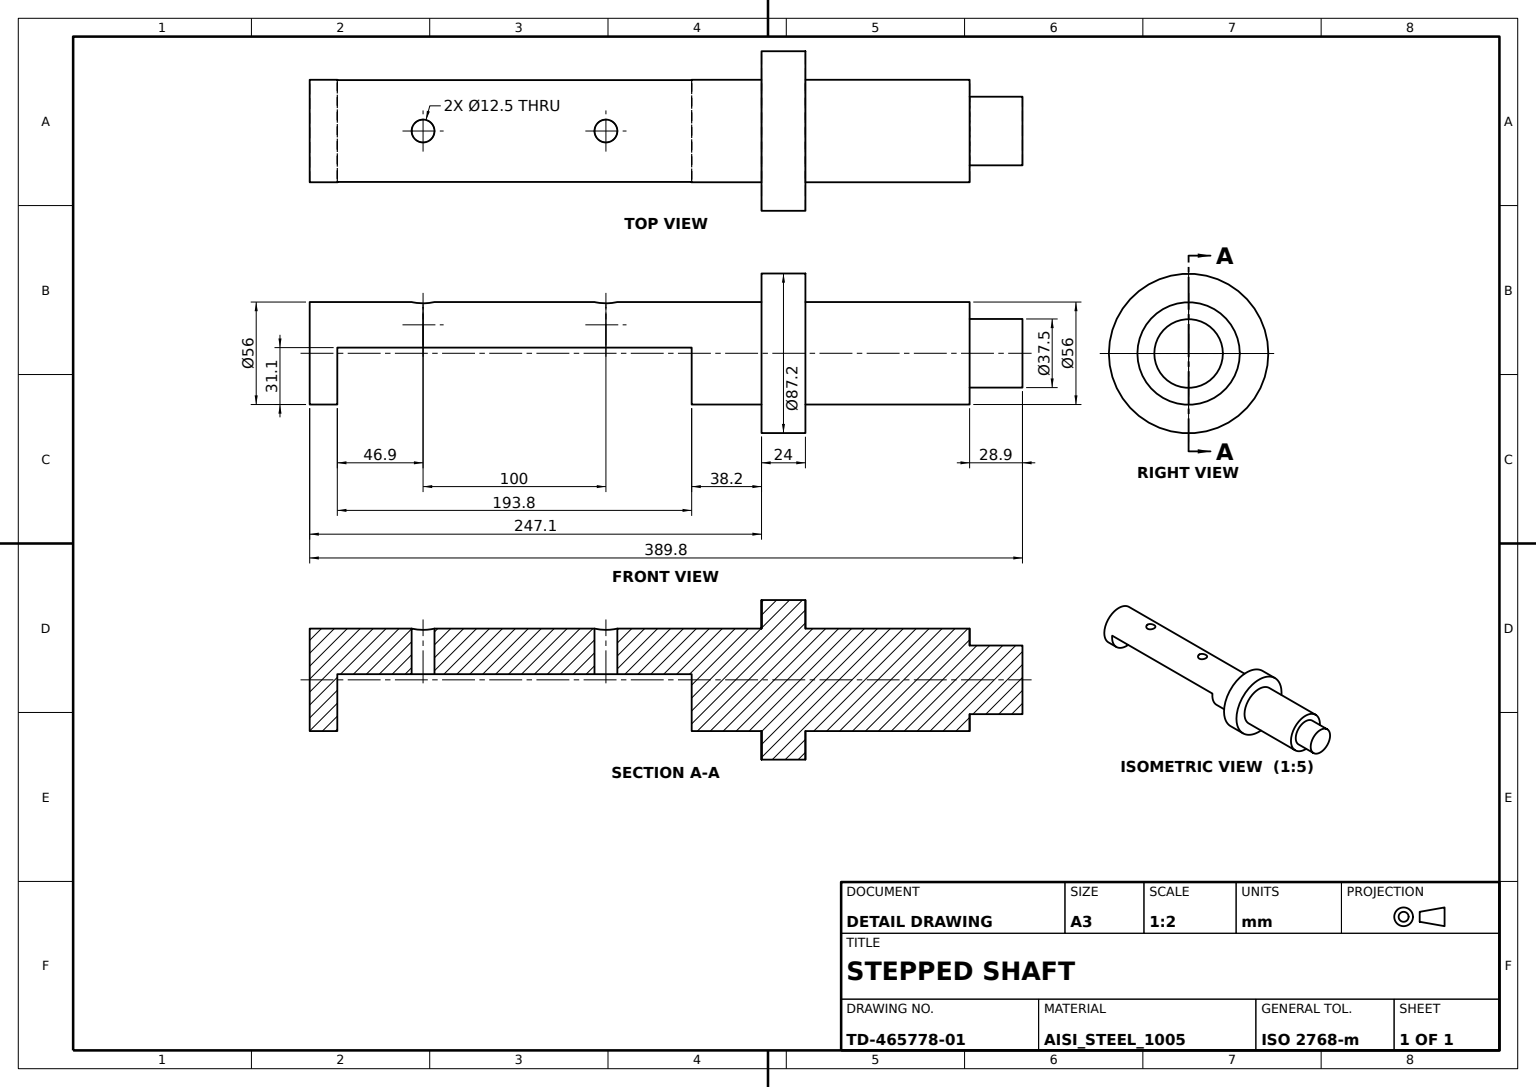
ISO-10303-21;
HEADER;
FILE_DESCRIPTION((''),'2;1');
FILE_NAME('','',(''),(''),'','','');
FILE_SCHEMA(('AUTOMOTIVE_DESIGN'));
ENDSEC;
DATA;
#1=APPLICATION_CONTEXT('');
#2=PRODUCT_CONTEXT('',#1,'mechanical');
#3=PRODUCT('','','',(#2));
#4=PRODUCT_DEFINITION_FORMATION('','',#3);
#5=PRODUCT_DEFINITION_CONTEXT('',#1,'design');
#6=PRODUCT_DEFINITION('','',#4,#5);
#7=PRODUCT_DEFINITION_SHAPE('','',#6);
#8=(LENGTH_UNIT()NAMED_UNIT(*)SI_UNIT(.MILLI.,.METRE.));
#9=(NAMED_UNIT(*)PLANE_ANGLE_UNIT()SI_UNIT($,.RADIAN.));
#10=(NAMED_UNIT(*)SI_UNIT($,.STERADIAN.)SOLID_ANGLE_UNIT());
#11=UNCERTAINTY_MEASURE_WITH_UNIT(LENGTH_MEASURE(0.005),#8,'distance_accuracy_value','');
#12=(GEOMETRIC_REPRESENTATION_CONTEXT(3)GLOBAL_UNCERTAINTY_ASSIGNED_CONTEXT((#11))GLOBAL_UNIT_ASSIGNED_CONTEXT((#8,#9,#10))REPRESENTATION_CONTEXT('',''));
#13=CARTESIAN_POINT('',(0.,18.75,142.7));
#14=VERTEX_POINT('',#13);
#15=CARTESIAN_POINT('',(0.,0.,142.7));
#16=DIRECTION('',(0.,0.,1.));
#17=DIRECTION('',(0.,1.,0.));
#18=AXIS2_PLACEMENT_3D('',#15,#16,#17);
#19=CIRCLE('',#18,18.75);
#20=EDGE_CURVE('',#14,#14,#19,.T.);
#21=ORIENTED_EDGE('',*,*,#20,.T.);
#22=EDGE_LOOP('',(#21));
#23=FACE_BOUND('',#22,.T.);
#24=DIRECTION('',(1.,0.,0.));
#25=AXIS2_PLACEMENT_3D('',#15,#16,#24);
#26=PLANE('',#25);
#27=ADVANCED_FACE('',(#23),#26,.T.);
#28=CARTESIAN_POINT('',(-28.,0.,-191.35));
#29=VERTEX_POINT('',#28);
#30=CARTESIAN_POINT('',(-27.923292,-2.470226,-191.018368));
#31=CARTESIAN_POINT('',(-28.038226,0.001909,-191.51522));
#32=CARTESIAN_POINT('',(-27.923806,2.462591,-191.020753));
#33=CARTESIAN_POINT('',(-27.649413,4.534425,-189.632288));
#34=CARTESIAN_POINT('',(-27.371989,5.92072,-187.562091));
#35=CARTESIAN_POINT('',(-27.254483,6.413877,-185.104449));
#36=CARTESIAN_POINT('',(-27.37134,5.923765,-182.643032));
#37=CARTESIAN_POINT('',(-27.649543,4.533953,-180.566538));
#38=CARTESIAN_POINT('',(-27.923952,2.461325,-179.178709));
#39=CARTESIAN_POINT('',(-28.037916,0.002745,-178.686152));
#40=CARTESIAN_POINT('',(-27.924382,-2.456758,-179.176687));
#41=CARTESIAN_POINT('',(-27.650228,-4.529699,-180.56301));
#42=CARTESIAN_POINT('',(-27.372311,-5.919433,-182.633271));
#43=CARTESIAN_POINT('',(-27.254354,-6.414385,-185.096275));
#44=CARTESIAN_POINT('',(-27.371534,-5.923021,-187.558096));
#45=CARTESIAN_POINT('',(-27.649072,-4.535591,-189.63023));
#46=B_SPLINE_CURVE_WITH_KNOTS('',3,(#30,#31,#32,#33,#34,#35,#36,#37,#38,#39,#40,#41,#42,#43,#44,#45,#30,#31,#32),.UNSPECIFIED.,.T.,.F.,(1,1,1,1,1,1,1,1,1,1,1,1,1,1,1,1,1,1,1,1,1,1,1),(-0.00734987,-0.004899913,-0.002449957,0.,0.002449957,0.004899913,0.00734987,0.009799826,0.012249783,0.014699739,0.017149696,0.019599653,0.022049609,0.024499566,0.026949522,0.029399479,0.031849436,0.034299392,0.036749349,0.039199305,0.041649262,0.044099218,0.046549175),.UNSPECIFIED.);
#47=EDGE_CURVE('',#29,#29,#46,.T.);
#48=ORIENTED_EDGE('',*,*,#47,.F.);
#49=EDGE_LOOP('',(#48));
#50=FACE_BOUND('',#49,.T.);
#51=CARTESIAN_POINT('',(-3.1,0.,-178.85));
#52=VERTEX_POINT('',#51);
#53=CARTESIAN_POINT('',(-3.1,0.,-185.1));
#54=AXIS2_PLACEMENT_3D('',#53,#24,#16);
#55=CIRCLE('',#54,6.25);
#56=EDGE_CURVE('',#52,#52,#55,.T.);
#57=ORIENTED_EDGE('',*,*,#56,.T.);
#58=EDGE_LOOP('',(#57));
#59=FACE_BOUND('',#58,.T.);
#60=CARTESIAN_POINT('',(-47.65,0.,-185.1));
#61=DIRECTION('',(0.,0.,-1.));
#62=AXIS2_PLACEMENT_3D('',#60,#24,#61);
#63=CYLINDRICAL_SURFACE('',#62,6.25);
#64=ADVANCED_FACE('',(#50,#59),#63,.F.);
#65=CARTESIAN_POINT('',(0.,18.75,113.8));
#66=VERTEX_POINT('',#65);
#67=CARTESIAN_POINT('',(0.,0.,113.8));
#68=AXIS2_PLACEMENT_3D('',#67,#16,#17);
#69=CIRCLE('',#68,18.75);
#70=EDGE_CURVE('',#66,#66,#69,.T.);
#71=ORIENTED_EDGE('',*,*,#70,.F.);
#72=EDGE_LOOP('',(#71));
#73=FACE_BOUND('',#72,.T.);
#74=CARTESIAN_POINT('',(0.,28.,113.8));
#75=VERTEX_POINT('',#74);
#76=CIRCLE('',#68,28.);
#77=EDGE_CURVE('',#75,#75,#76,.T.);
#78=ORIENTED_EDGE('',*,*,#77,.T.);
#79=EDGE_LOOP('',(#78));
#80=FACE_BOUND('',#79,.T.);
#81=AXIS2_PLACEMENT_3D('',#67,#16,#24);
#82=PLANE('',#81);
#83=ADVANCED_FACE('',(#73,#80),#82,.T.);
#84=CARTESIAN_POINT('',(0.,28.,24.));
#85=VERTEX_POINT('',#84);
#86=CARTESIAN_POINT('',(0.,0.,24.));
#87=AXIS2_PLACEMENT_3D('',#86,#16,#17);
#88=CIRCLE('',#87,28.);
#89=EDGE_CURVE('',#85,#85,#88,.T.);
#90=ORIENTED_EDGE('',*,*,#89,.F.);
#91=EDGE_LOOP('',(#90));
#92=FACE_BOUND('',#91,.T.);
#93=CARTESIAN_POINT('',(0.,43.6,24.));
#94=VERTEX_POINT('',#93);
#95=CIRCLE('',#87,43.6);
#96=EDGE_CURVE('',#94,#94,#95,.T.);
#97=ORIENTED_EDGE('',*,*,#96,.T.);
#98=EDGE_LOOP('',(#97));
#99=FACE_BOUND('',#98,.T.);
#100=AXIS2_PLACEMENT_3D('',#86,#16,#24);
#101=PLANE('',#100);
#102=ADVANCED_FACE('',(#92,#99),#101,.T.);
#103=ORIENTED_EDGE('',*,*,#96,.F.);
#104=EDGE_LOOP('',(#103));
#105=FACE_BOUND('',#104,.T.);
#106=CARTESIAN_POINT('',(0.,43.6,0.));
#107=VERTEX_POINT('',#106);
#108=CARTESIAN_POINT('',(0.,0.,0.));
#109=AXIS2_PLACEMENT_3D('',#108,#16,#17);
#110=CIRCLE('',#109,43.6);
#111=EDGE_CURVE('',#107,#107,#110,.T.);
#112=ORIENTED_EDGE('',*,*,#111,.T.);
#113=EDGE_LOOP('',(#112));
#114=FACE_BOUND('',#113,.T.);
#115=DIRECTION('',(-1.,0.,0.));
#116=AXIS2_PLACEMENT_3D('',#86,#61,#115);
#117=CYLINDRICAL_SURFACE('',#116,43.6);
#118=ADVANCED_FACE('',(#105,#114),#117,.T.);
#119=ORIENTED_EDGE('',*,*,#70,.T.);
#120=EDGE_LOOP('',(#119));
#121=FACE_BOUND('',#120,.T.);
#122=ORIENTED_EDGE('',*,*,#20,.F.);
#123=EDGE_LOOP('',(#122));
#124=FACE_BOUND('',#123,.T.);
#125=AXIS2_PLACEMENT_3D('',#15,#61,#115);
#126=CYLINDRICAL_SURFACE('',#125,18.75);
#127=ADVANCED_FACE('',(#121,#124),#126,.T.);
#128=ORIENTED_EDGE('',*,*,#77,.F.);
#129=EDGE_LOOP('',(#128));
#130=FACE_BOUND('',#129,.T.);
#131=ORIENTED_EDGE('',*,*,#89,.T.);
#132=EDGE_LOOP('',(#131));
#133=FACE_BOUND('',#132,.T.);
#134=AXIS2_PLACEMENT_3D('',#67,#61,#115);
#135=CYLINDRICAL_SURFACE('',#134,28.);
#136=ADVANCED_FACE('',(#130,#133),#135,.T.);
#137=CARTESIAN_POINT('',(-3.1,-27.827864,-232.));
#138=VERTEX_POINT('',#137);
#139=CARTESIAN_POINT('',(-3.1,27.827864,-232.));
#140=VERTEX_POINT('',#139);
#141=CARTESIAN_POINT('',(0.,0.,-232.));
#142=AXIS2_PLACEMENT_3D('',#141,#61,#115);
#143=CIRCLE('',#142,28.);
#144=EDGE_CURVE('',#138,#140,#143,.F.);
#145=ORIENTED_EDGE('',*,*,#144,.T.);
#146=CARTESIAN_POINT('',(-3.1,28.9,-232.));
#147=DIRECTION('',(0.,-1.,0.));
#148=VECTOR('',#147,1000.);
#149=LINE('',#146,#148);
#150=EDGE_CURVE('',#138,#140,#149,.F.);
#151=ORIENTED_EDGE('',*,*,#150,.F.);
#152=EDGE_LOOP('',(#145,#151));
#153=FACE_BOUND('',#152,.T.);
#154=AXIS2_PLACEMENT_3D('',#146,#61,#115);
#155=PLANE('',#154);
#156=ADVANCED_FACE('',(#153),#155,.F.);
#157=CARTESIAN_POINT('',(0.,28.,-247.1));
#158=VERTEX_POINT('',#157);
#159=CARTESIAN_POINT('',(0.,0.,-247.1));
#160=AXIS2_PLACEMENT_3D('',#159,#16,#17);
#161=CIRCLE('',#160,28.);
#162=EDGE_CURVE('',#158,#158,#161,.T.);
#163=ORIENTED_EDGE('',*,*,#162,.F.);
#164=EDGE_LOOP('',(#163));
#165=FACE_BOUND('',#164,.T.);
#166=AXIS2_PLACEMENT_3D('',#159,#16,#24);
#167=PLANE('',#166);
#168=ADVANCED_FACE('',(#165),#167,.F.);
#169=CARTESIAN_POINT('',(-3.1,-27.827864,-38.2));
#170=VERTEX_POINT('',#169);
#171=CARTESIAN_POINT('',(-3.1,27.827864,-38.2));
#172=VERTEX_POINT('',#171);
#173=CARTESIAN_POINT('',(-3.1,28.9,-38.2));
#174=LINE('',#173,#148);
#175=EDGE_CURVE('',#170,#172,#174,.F.);
#176=ORIENTED_EDGE('',*,*,#175,.T.);
#177=CARTESIAN_POINT('',(0.,0.,-38.2));
#178=AXIS2_PLACEMENT_3D('',#177,#16,#24);
#179=CIRCLE('',#178,28.);
#180=EDGE_CURVE('',#172,#170,#179,.F.);
#181=ORIENTED_EDGE('',*,*,#180,.T.);
#182=EDGE_LOOP('',(#176,#181));
#183=FACE_BOUND('',#182,.T.);
#184=CARTESIAN_POINT('',(35.85,28.9,-38.2));
#185=AXIS2_PLACEMENT_3D('',#184,#16,#24);
#186=PLANE('',#185);
#187=ADVANCED_FACE('',(#183),#186,.F.);
#188=CARTESIAN_POINT('',(-28.,0.,-91.35));
#189=VERTEX_POINT('',#188);
#190=CARTESIAN_POINT('',(-27.923292,-2.470226,-91.018368));
#191=CARTESIAN_POINT('',(-28.038226,0.001909,-91.51522));
#192=CARTESIAN_POINT('',(-27.923806,2.462591,-91.020753));
#193=CARTESIAN_POINT('',(-27.649413,4.534425,-89.632288));
#194=CARTESIAN_POINT('',(-27.371989,5.92072,-87.562091));
#195=CARTESIAN_POINT('',(-27.254483,6.413877,-85.104449));
#196=CARTESIAN_POINT('',(-27.37134,5.923765,-82.643032));
#197=CARTESIAN_POINT('',(-27.649543,4.533953,-80.566538));
#198=CARTESIAN_POINT('',(-27.923952,2.461325,-79.178709));
#199=CARTESIAN_POINT('',(-28.037916,0.002745,-78.686152));
#200=CARTESIAN_POINT('',(-27.924382,-2.456758,-79.176687));
#201=CARTESIAN_POINT('',(-27.650228,-4.529699,-80.56301));
#202=CARTESIAN_POINT('',(-27.372311,-5.919433,-82.633271));
#203=CARTESIAN_POINT('',(-27.254354,-6.414385,-85.096275));
#204=CARTESIAN_POINT('',(-27.371534,-5.923021,-87.558096));
#205=CARTESIAN_POINT('',(-27.649072,-4.535591,-89.63023));
#206=B_SPLINE_CURVE_WITH_KNOTS('',3,(#190,#191,#192,#193,#194,#195,#196,#197,#198,#199,#200,#201,#202,#203,#204,#205,#190,#191,#192),.UNSPECIFIED.,.T.,.F.,(1,1,1,1,1,1,1,1,1,1,1,1,1,1,1,1,1,1,1,1,1,1,1),(-0.00734987,-0.004899913,-0.002449957,0.,0.002449957,0.004899913,0.00734987,0.009799826,0.012249783,0.014699739,0.017149696,0.019599653,0.022049609,0.024499566,0.026949522,0.029399479,0.031849436,0.034299392,0.036749349,0.039199305,0.041649262,0.044099218,0.046549175),.UNSPECIFIED.);
#207=EDGE_CURVE('',#189,#189,#206,.T.);
#208=ORIENTED_EDGE('',*,*,#207,.F.);
#209=EDGE_LOOP('',(#208));
#210=FACE_BOUND('',#209,.T.);
#211=CARTESIAN_POINT('',(-3.1,0.,-78.85));
#212=VERTEX_POINT('',#211);
#213=CARTESIAN_POINT('',(-3.1,0.,-85.1));
#214=AXIS2_PLACEMENT_3D('',#213,#24,#16);
#215=CIRCLE('',#214,6.25);
#216=EDGE_CURVE('',#212,#212,#215,.T.);
#217=ORIENTED_EDGE('',*,*,#216,.T.);
#218=EDGE_LOOP('',(#217));
#219=FACE_BOUND('',#218,.T.);
#220=CARTESIAN_POINT('',(-47.65,0.,-85.1));
#221=AXIS2_PLACEMENT_3D('',#220,#24,#61);
#222=CYLINDRICAL_SURFACE('',#221,6.25);
#223=ADVANCED_FACE('',(#210,#219),#222,.F.);
#224=ORIENTED_EDGE('',*,*,#207,.T.);
#225=EDGE_LOOP('',(#224));
#226=FACE_BOUND('',#225,.T.);
#227=ORIENTED_EDGE('',*,*,#162,.T.);
#228=EDGE_LOOP('',(#227));
#229=FACE_BOUND('',#228,.T.);
#230=CARTESIAN_POINT('',(0.,28.,0.));
#231=VERTEX_POINT('',#230);
#232=CIRCLE('',#109,28.);
#233=EDGE_CURVE('',#231,#231,#232,.T.);
#234=ORIENTED_EDGE('',*,*,#233,.F.);
#235=EDGE_LOOP('',(#234));
#236=FACE_BOUND('',#235,.T.);
#237=ORIENTED_EDGE('',*,*,#47,.T.);
#238=EDGE_LOOP('',(#237));
#239=FACE_BOUND('',#238,.T.);
#240=CARTESIAN_POINT('',(-3.1,-27.827864,-247.1));
#241=VECTOR('',#16,1000.);
#242=LINE('',#240,#241);
#243=EDGE_CURVE('',#170,#138,#242,.F.);
#244=ORIENTED_EDGE('',*,*,#243,.F.);
#245=ORIENTED_EDGE('',*,*,#180,.F.);
#246=CARTESIAN_POINT('',(-3.1,27.827864,-247.1));
#247=LINE('',#246,#241);
#248=EDGE_CURVE('',#140,#172,#247,.T.);
#249=ORIENTED_EDGE('',*,*,#248,.F.);
#250=ORIENTED_EDGE('',*,*,#144,.F.);
#251=EDGE_LOOP('',(#244,#245,#249,#250));
#252=FACE_BOUND('',#251,.T.);
#253=CYLINDRICAL_SURFACE('',#166,28.);
#254=ADVANCED_FACE('',(#226,#229,#236,#239,#252),#253,.T.);
#255=ORIENTED_EDGE('',*,*,#56,.F.);
#256=EDGE_LOOP('',(#255));
#257=FACE_BOUND('',#256,.T.);
#258=ORIENTED_EDGE('',*,*,#248,.T.);
#259=ORIENTED_EDGE('',*,*,#175,.F.);
#260=ORIENTED_EDGE('',*,*,#243,.T.);
#261=ORIENTED_EDGE('',*,*,#150,.T.);
#262=EDGE_LOOP('',(#258,#259,#260,#261));
#263=FACE_BOUND('',#262,.T.);
#264=ORIENTED_EDGE('',*,*,#216,.F.);
#265=EDGE_LOOP('',(#264));
#266=FACE_BOUND('',#265,.T.);
#267=AXIS2_PLACEMENT_3D('',#173,#115,#16);
#268=PLANE('',#267);
#269=ADVANCED_FACE('',(#257,#263,#266),#268,.F.);
#270=ORIENTED_EDGE('',*,*,#111,.F.);
#271=EDGE_LOOP('',(#270));
#272=FACE_BOUND('',#271,.T.);
#273=ORIENTED_EDGE('',*,*,#233,.T.);
#274=EDGE_LOOP('',(#273));
#275=FACE_BOUND('',#274,.T.);
#276=AXIS2_PLACEMENT_3D('',#108,#16,#24);
#277=PLANE('',#276);
#278=ADVANCED_FACE('',(#272,#275),#277,.F.);
#279=CLOSED_SHELL('',(#27,#64,#83,#102,#118,#127,#136,#156,#168,#187,#223,#254,#269,#278));
#280=MANIFOLD_SOLID_BREP('',#279);
#281=ADVANCED_BREP_SHAPE_REPRESENTATION('',(#280),#12);
#282=SHAPE_DEFINITION_REPRESENTATION(#7,#281);
ENDSEC;
END-ISO-10303-21;
